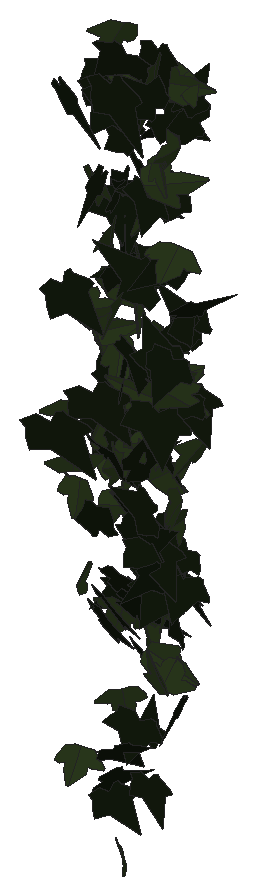
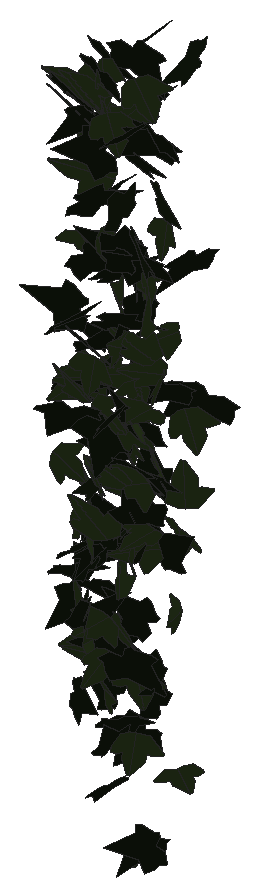
# SketchUp Ruby script. Lengths in inches.
U = 1.inch
M = Sketchup.active_model
def pt(a) = Geom::Point3d.new(a.map { |v| v * U })
def face(e, loops, mat)
  f = e.add_face(loops[0].map { |a| pt(a) })
  loops[1..].each { |l| e.add_face(l.map { |a| pt(a) }).erase! }
  f.material = f.back_material = mat if mat
  f
end
# faces: each face lists its corners as indices into pts; further lists are holes
def faces(e, pts, list, mat = nil) = list.each { |f| face(e, (f[0].is_a?(Array) ? f : [f]).map { |l| l.map { |i| pts[i] } }, mat) }
# xy, xz, yz: faces in a plane at the given z, y or x. An outline is a flat list of corners, or four numbers for a rectangle; further outlines are holes
def ring(l) = l.size == 4 ? [[l[0], l[1]], [l[2], l[1]], [l[2], l[3]], [l[0], l[3]]] : l.each_slice(2).to_a
def flat(e, list, mat, &to3) = list.each { |f| face(e, (f[0].is_a?(Array) ? f : [f]).map { |l| ring(l).map { |u, v| to3.(u, v) } }, mat) }
def xy(e, z, list, mat = nil) = flat(e, list, mat) { |x, y| [x, y, z] }
def xz(e, y, list, mat = nil) = flat(e, list, mat) { |x, z| [x, y, z] }
def yz(e, x, list, mat = nil) = flat(e, list, mat) { |y, z| [x, y, z] }
def lines(e, pts, list) = list.each { |a, b| e.add_line(pt(pts[a]), pt(pts[b])) }
# prism: a flat outline (further loops are holes) pulled along v
def prism(e, loops, v, mat = nil)
  f = face(e, loops, mat); d = Geom::Vector3d.new(v.map { |x| x * U })
  f.pushpull(f.normal.samedirection?(d) ? d.length : -d.length)
end
def box(e, o, s, mat = nil) = prism(e, [[o, [o[0] + s[0], o[1], o[2]], [o[0] + s[0], o[1] + s[1], o[2]], [o[0], o[1] + s[1], o[2]]]], [0, 0, s[2]], mat)
def at(x, y, z, deg = 0) = Geom::Transformation.translation(pt([x, y, z])) * Geom::Transformation.rotation(ORIGIN, Z_AXIS, deg.degrees)
def axes(o, x, y, z) = Geom::Transformation.new([*x, 0, *y, 0, *z, 0, *pt(o).to_a, 1])
def part(name) = M.definitions.add(name)
# library, detail: a bought-in or finely detailed component or shape, given as its bounding box
def library(name, o, s) = part(name).tap { |d| box(d.entities, o, s) }
def detail(e, o, s) = box(e.add_group.entities, o, s)
def put(e, d, t, mat = nil) = e.add_instance(d, t).tap { |i| i.material = mat if mat }
def group(e, t, mat = nil) = e.add_group.tap { |g| g.transformation = t; g.material = mat if mat }.entities
root = M.entities
M.materials.add("1026 AP 7946 SUNNY SIDE UP").color = [254, 231, 186]
M.materials.add("efeu1").color = [18, 25, 13]
M.materials.add("efeu2").color = [43, 57, 29]
c1 = part("ivyleaf_9")
p = [[1.54,2.16,1.25],[1.36,2.04,1.19],[-0.21,0.99,0.68],[-0.71,1.11,0.82],[-0.85,0.86,0.67],[-0.8,0.17,0.21],
  [-0.9,-0.01,0.1],[-0.67,-0.16,-0.02],[-0.08,-0.08,-0.05],[-0.03,-0.6,-0.4],[0.65,-0.88,-0.66],[0.83,-0.6,-0.49],
  [1.29,-0.42,-0.43],[1.8125,-0.07,-0.26],[1.21,0.44,0.15]]
faces(c1.entities,p,[[0,1,2,3,4,5,6,7,8,9,10,11,12,13,14]],"efeu1")
c2 = part("ivyleaf_10")
p = [[0,0.5,-0.03],[-0.0625,2.02,-0.43],[-0.19,2.01,-0.46],[-0.54,1.05,-0.29],[-0.52,0.625,-0.18],[-0.83,0.76,-0.28],
  [-1.16,0.64,-0.33],[-1.15,0.33,-0.24],[-0.77,-0.39,0.02],[-0.3,-0.51,0.16],[0.04,-0.48,0.23],[-0.02,2.01,-0.4375],
  [-0.06,2.01,-0.43],[0.04,-0.49,0.23],[0.67,-0.49,0.14],[1.38,0.36,-0.2],[1.375,0.51,-0.24],[0.81,0.65,-0.19],
  [0.62,0.59,-0.15],[0.6,1.09,-0.28],[0.5,1.23,-0.31]]
faces(c2.entities,p,[[0,1,2,3,4,5,6,7,8,9,10],[11,12,0,13,14,15,16,17,18,19,20]],"efeu2")
put(root,c1,axes([117.89,209.16,260.61],[-0.12502,-0.13654,-0.30499],[0.32147,0.21547,-0.1581],[0.39789,-0.21699,0.0319]),"1026 AP 7946 SUNNY SIDE UP")
put(root,c1,axes([118.01,209.3,267.36],[0.35139,-0.25579,-0.05878],[-0.08033,0.02908,-0.34919],[0.40368,0.22845,-0.01832]),"1026 AP 7946 SUNNY SIDE UP")
put(root,c1,axes([118.04,209.3,263.4],[0.10905,-0.2297,-0.2487],[-0.06595,0.23727,-0.24493],[0.51831,0.07852,0.02116]),"1026 AP 7946 SUNNY SIDE UP")
put(root,c1,axes([118.89,209.58,267.58],[0.16751,-0.3674,-0.0775],[-0.0277,0.07105,-0.39365],[0.58838,0.10794,0.00353]),"1026 AP 7946 SUNNY SIDE UP")
put(root,c1,axes([119.68,209.67,259.19],[0.02681,-0.30366,-0.03755],[0.03363,-0.03351,0.31249],[-0.4794,-0.01933,0.01982]),"1026 AP 7946 SUNNY SIDE UP")
put(root,c2,axes([117.7,209.92,260.55],[-0.22825,-0.27044,0.05167],[-0.01496,-0.05347,-0.31605],[0.43268,-0.14451,0.01633]),"1026 AP 7946 SUNNY SIDE UP")
put(root,c2,axes([118.62,210.08,262.89],[0.1701,-0.19875,0.2303],[0.12167,-0.21227,-0.23307],[0.45571,0.13086,-0.02374]),"1026 AP 7946 SUNNY SIDE UP")
put(root,c1,axes([118.25,209.89,261.01],[-0.0783,-0.2007,-0.24489],[0.20388,0.20421,-0.2054],[0.44317,-0.1294,0.05123]),"1026 AP 7946 SUNNY SIDE UP")
put(root,c2,axes([117.79,210.02,253.51],[0.28029,0.19308,-0.09406],[-0.07953,-0.07884,-0.27072],[-0.32705,0.18465,-0.01478]),"1026 AP 7946 SUNNY SIDE UP")
put(root,c1,axes([119.51,210.12,257.75],[-0.0668,0.06136,-0.27059],[0.09308,-0.25765,-0.07329],[-0.41433,-0.06777,0.02716]),"1026 AP 7946 SUNNY SIDE UP")
put(root,c1,axes([118.29,210.23,266.77],[-0.1118,-0.21782,0.17072],[-0.07074,-0.16088,-0.23692],[0.4257,-0.08394,0.00547]),"1026 AP 7946 SUNNY SIDE UP")
put(root,c1,axes([118.72,209.88,253.97],[0.27527,0.19906,0.05238],[0.06943,0.02727,-0.2725],[-0.31506,0.17993,-0.01429]),"1026 AP 7946 SUNNY SIDE UP")
put(root,c2,axes([119.66,210,255.55],[-0.30115,0.16584,-0.13563],[-0.13467,0.10306,0.26083],[0.3055,0.20891,-0.01872]),"1026 AP 7946 SUNNY SIDE UP")
put(root,c1,axes([119.43,210.22,260.87],[-0.19506,-0.27654,-0.09752],[0.07322,0.0811,-0.31164],[0.45293,-0.13221,0.00838]),"1026 AP 7946 SUNNY SIDE UP")
put(root,c2,axes([118.65,210.2,251.55],[-0.21172,0.17466,0.14632],[0.15877,-0.09978,0.22601],[0.31528,0.16753,-0.01555]),"1026 AP 7946 SUNNY SIDE UP")
put(root,c1,axes([119.29,210.2,258.15],[-0.07414,-0.25428,-0.16502],[0.10957,0.147,-0.26304],[0.45844,-0.07625,0.03618]),"1026 AP 7946 SUNNY SIDE UP")
put(root,c1,axes([119.47,210.03,267.21],[-0.12137,0.13688,0.25052],[-0.22034,0.19825,-0.16013],[-0.37822,-0.15941,0.0129]),"1026 AP 7946 SUNNY SIDE UP")
put(root,c2,axes([117.53,210.24,259.18],[-0.30253,-0.25451,-0.03509],[-0.05348,-0.01511,0.32808],[-0.39991,0.19456,-0.01733]),"1026 AP 7946 SUNNY SIDE UP")
put(root,c1,axes([118.77,210.4375,261.6875],[-0.02303,-0.23728,0.2184],[0.05144,-0.21356,-0.24363],[0.4991,0.01106,0.03519]),"1026 AP 7946 SUNNY SIDE UP")
put(root,c2,axes([119.13,210.28,261.125],[-0.13156,-0.04352,-0.27512],[-0.41464,-0.04835,0.09303],[-0.09359,0.27541,-0.02544]),"1026 AP 7946 SUNNY SIDE UP")
put(root,c1,axes([118.91,210.27,258.09],[-0.06697,0.0593,0.29108],[0.32388,-0.19339,0.07276],[0.31734,0.20989,-0.01283]),"1026 AP 7946 SUNNY SIDE UP")
put(root,c1,axes([119.625,210.36,261.95],[-0.39019,-0.07568,-0.12099],[0.19163,-0.00194,-0.26496],[0.10628,-0.27435,0.03352]),"1026 AP 7946 SUNNY SIDE UP")
put(root,c2,axes([118.77,210.34,259.96],[0.37069,-0.14453,0.05282],[0.05077,-0.04667,-0.28421],[0.23618,0.23688,-0.02181]),"1026 AP 7946 SUNNY SIDE UP")
put(root,c1,axes([118.83,210.42,254.35],[-0.23868,-0.21538,-0.01707],[0.03451,0.00327,-0.27093],[0.33777,-0.15253,0.01562]),"1026 AP 7946 SUNNY SIDE UP")
put(root,c1,axes([117.96,210.41,265.07],[-0.30032,0.07525,-0.25163],[0.3196,-0.14102,-0.20895],[-0.24471,-0.27652,0.03593]),"1026 AP 7946 SUNNY SIDE UP")
put(root,c1,axes([118.46,210.49,261.52],[-0.11282,-0.02764,-0.27999],[0.37587,-0.14206,-0.05099],[-0.20744,-0.24238,0.05988]),"1026 AP 7946 SUNNY SIDE UP")
put(root,c1,axes([118.98,210.07,259.69],[0.05149,0.07369,0.32786],[0.34732,0.23008,-0.07705],[-0.37756,0.22171,-0.02617]),"1026 AP 7946 SUNNY SIDE UP")
put(root,c1,axes([118.57,210.34,267.8],[0.18066,0.0622,-0.2606],[-0.31294,-0.15802,-0.13389],[-0.26511,0.22891,-0.01954]),"1026 AP 7946 SUNNY SIDE UP")
put(root,c2,axes([117.41,210.45,258.625],[0.3814,-0.10016,0.0848],[0.10439,-0.05542,-0.26947],[0.17575,0.25027,-0.02396]),"1026 AP 7946 SUNNY SIDE UP")
put(root,c1,axes([118.03,210.53,259.34],[0.43236,-0.16438,-0.07785],[0.13355,-0.0022,0.32735],[-0.25049,-0.2849,0.04017]),"1026 AP 7946 SUNNY SIDE UP")
put(root,c1,axes([118.94,210.6,264.97],[-0.08326,-0.25512,0.11036],[-0.02691,-0.10732,-0.26901],[0.43514,-0.05545,0.00448]),"1026 AP 7946 SUNNY SIDE UP")
put(root,c1,axes([119.01,210.54,263.21],[-0.23748,-0.30417,-0.03617],[-0.04349,-0.02351,0.34941],[-0.47918,0.15288,-0.01379]),"1026 AP 7946 SUNNY SIDE UP")
put(root,c2,axes([119.45,210.39,255.4],[0.40233,0.02742,-0.07135],[0.10307,0.03597,0.26377],[0.05611,-0.26267,0.02709]),"1026 AP 7946 SUNNY SIDE UP")
put(root,c2,axes([119.1,210.58,265.6875],[0.22542,-0.09301,0.23138],[0.30146,-0.11805,-0.17671],[0.23626,0.23937,0.00471]),"1026 AP 7946 SUNNY SIDE UP")
put(root,c2,axes([119.4,210.66,266.02],[-0.01006,0.0395,0.29127],[0.12409,-0.27131,0.03933],[0.43104,0.07903,-0.00452]),"1026 AP 7946 SUNNY SIDE UP")
put(root,c1,axes([117.92,210.39,258.01],[0.11424,-0.07137,0.30027],[-0.26332,0.23971,0.10473],[-0.39229,-0.18169,0.01714]),"1026 AP 7946 SUNNY SIDE UP")
put(root,c2,axes([117.65,210.28,256.84],[0.058,-0.03851,0.26789],[-0.18245,0.23348,0.0539],[-0.37128,-0.12075,0.01537]),"1026 AP 7946 SUNNY SIDE UP")
put(root,c2,axes([119.66,210.43,259.04],[0.21606,-0.27018,-0.13536],[-0.08771,0.11731,-0.31156],[0.46312,0.14826,0.00414]),"1026 AP 7946 SUNNY SIDE UP")
put(root,c1,axes([119.25,210.64,257.0625],[-0.36078,-0.1331,-0.0337],[0.06211,-0.00466,-0.2722],[0.20608,-0.23162,0.02304]),"1026 AP 7946 SUNNY SIDE UP")
put(root,c1,axes([118.93,210.59,253.1],[0.02293,-0.25363,-0.04997],[-0.00682,0.04689,-0.26144],[0.40556,0.01513,-0.00157]),"1026 AP 7946 SUNNY SIDE UP")
put(root,c2,axes([117.74,210.32,262.38],[0.00162,-0.04504,-0.30723],[0.23296,0.25956,-0.03837],[0.41264,-0.14636,0.02286]),"1026 AP 7946 SUNNY SIDE UP")
put(root,c2,axes([119.02,210.75,260],[-0.04851,0.03994,0.30529],[-0.06276,-0.29557,0.03506],[0.46562,-0.03568,0.03653]),"1026 AP 7946 SUNNY SIDE UP")
put(root,c2,axes([119.18,210.49,255.76],[0.17065,0.06931,0.28511],[0.41197,0.09192,-0.12921],[-0.17602,0.28232,-0.026]),"1026 AP 7946 SUNNY SIDE UP")
put(root,c2,axes([118.11,210.73,259.15],[-0.07921,0.10847,0.27956],[0.15036,-0.25343,0.12144],[0.43327,0.10778,0.00896]),"1026 AP 7946 SUNNY SIDE UP")
put(root,c1,axes([119.32,210.54,261.72],[-0.30706,-0.17895,0.10986],[0.10631,0.08528,0.27287],[-0.31069,0.20604,-0.01521]),"1026 AP 7946 SUNNY SIDE UP")
put(root,c1,axes([119.3,210.78,263.65],[-0.02249,0.00095,-0.29261],[0.04815,-0.28274,-0.00421],[-0.44403,-0.03071,0.01436]),"1026 AP 7946 SUNNY SIDE UP")
put(root,c1,axes([119.41,210.8,256.33],[-0.0398,-0.07219,0.25686],[-0.04798,-0.24837,-0.0786],[0.40595,-0.03643,0.0159]),"1026 AP 7946 SUNNY SIDE UP")
put(root,c2,axes([117.72,210.6,259.65],[0.27195,-0.21842,-0.0076],[0.02796,0.00627,0.28647],[-0.34244,-0.17295,0.01735]),"1026 AP 7946 SUNNY SIDE UP")
put(root,c2,axes([119.43,210.67,263.9375],[0.3982,0.10783,-0.08347],[-0.10153,-0.05588,-0.28271],[-0.18686,0.26014,-0.02427]),"1026 AP 7946 SUNNY SIDE UP")
put(root,c1,axes([119.52,210.77,254.8125],[-0.16421,0.07154,-0.25283],[0.26209,-0.18253,-0.12874],[-0.30558,-0.195,0.02545]),"1026 AP 7946 SUNNY SIDE UP")
put(root,c1,axes([119.58,210.79,257.33],[-0.24316,-0.23222,-0.00877],[0.0253,-0.00208,-0.28704],[0.36444,-0.15479,0.01407]),"1026 AP 7946 SUNNY SIDE UP")
put(root,c2,axes([118.18,210.71,261.45],[0.19102,0.26514,-0.10917],[-0.0497,-0.10361,-0.30073],[-0.4471,0.1248,-0.01321]),"1026 AP 7946 SUNNY SIDE UP")
put(root,c2,axes([118.27,210.84,260.54],[-0.06525,-0.1992,0.18117],[-0.05361,-0.17368,-0.21063],[0.41556,-0.05368,0.00127]),"1026 AP 7946 SUNNY SIDE UP")
put(root,c1,axes([119.53,210.87,261.02],[-0.32071,-0.17503,0.02733],[-0.01203,-0.03324,-0.2763],[0.27834,-0.20311,0.01955]),"1026 AP 7946 SUNNY SIDE UP")
put(root,c2,axes([119.4,210.6,261.11],[-0.25221,-0.16823,-0.26059],[0.31878,0.15231,-0.23679],[0.35406,-0.25697,0.02757]),"1026 AP 7946 SUNNY SIDE UP")
put(root,c1,axes([117.97,210.77,256.78],[0.32068,0.01393,-0.16905],[0.25102,0.04795,0.20876],[0.06413,-0.25738,0.02818]),"1026 AP 7946 SUNNY SIDE UP")
put(root,c1,axes([118.17,210.72,258.42],[0.45091,-0.14505,-0.03748],[-0.06549,-0.00374,-0.33031],[0.22552,0.28894,-0.02098]),"1026 AP 7946 SUNNY SIDE UP")
put(root,c1,axes([118.85,210.63,253.93],[-0.15939,-0.10615,0.21857],[0.21106,0.16537,0.15184],[-0.30861,0.16792,-0.00904]),"1026 AP 7946 SUNNY SIDE UP")
put(root,c2,axes([117.68,210.73,261.7],[-0.12905,0.26484,-0.02049],[-0.00297,-0.02298,-0.28564],[-0.41779,-0.08165,0.00836]),"1026 AP 7946 SUNNY SIDE UP")
put(root,c2,axes([119.06,210.63,265.24],[0.14067,0.01624,-0.33931],[0.47847,0.12771,0.09236],[0.20022,-0.3166,0.01769]),"1026 AP 7946 SUNNY SIDE UP")
put(root,c1,axes([119.45,210.97,257.8],[-0.15824,-0.2005,0.12695],[-0.05739,-0.12035,-0.23101],[0.36652,-0.10541,0.01863]),"1026 AP 7946 SUNNY SIDE UP")
put(root,c2,axes([119.35,210.98,258.33],[-0.00053,-0.02027,-0.27346],[-0.06297,-0.26231,0.01916],[-0.41366,0.03996,-0.00257]),"1026 AP 7946 SUNNY SIDE UP")
put(root,c2,axes([118.89,210.75,267.46],[0.01018,-0.3284,-0.10986],[0.03146,0.10497,-0.33707],[0.5411,0.00007,0.02166]),"1026 AP 7946 SUNNY SIDE UP")
put(root,c2,axes([118.76,210.85,266.68],[0.12519,-0.28067,0.02869],[0.00089,-0.03043,-0.30062],[0.44374,0.07924,-0.00749]),"1026 AP 7946 SUNNY SIDE UP")
put(root,c1,axes([118.43,210.71,265.96],[-0.29493,-0.01829,-0.2132],[-0.32651,0.01475,0.19272],[-0.00207,0.27883,-0.02253]),"1026 AP 7946 SUNNY SIDE UP")
put(root,c1,axes([117.84,210.91,259.8],[-0.36309,-0.09377,-0.08664],[0.13455,0.0106,-0.25576],[0.14459,-0.24534,0.02042]),"1026 AP 7946 SUNNY SIDE UP")
put(root,c2,axes([118.27,210.82,266.79],[0.22731,0.21344,0.10504],[-0.11283,-0.0728,0.26454],[0.35355,-0.16046,0.01689]),"1026 AP 7946 SUNNY SIDE UP")
put(root,c2,axes([117.57,210.76,264.76],[-0.34906,0.15718,0.04591],[-0.0782,0.00503,-0.27906],[-0.2443,-0.22619,0.02374]),"1026 AP 7946 SUNNY SIDE UP")
put(root,c2,axes([117.89,210.77,263.83],[0.03254,-0.30122,-0.10367],[0.02109,0.09987,-0.30983],[0.49807,0.01545,0.01989]),"1026 AP 7946 SUNNY SIDE UP")
put(root,c2,axes([118.34,210.95,262.5],[-0.08891,0.21599,-0.22142],[0.08243,-0.20971,-0.23123],[-0.47337,-0.07709,0.00132]),"1026 AP 7946 SUNNY SIDE UP")
put(root,c1,axes([118.66,211,258.1],[0.33461,-0.09722,-0.18923],[0.28017,-0.04844,0.23951],[-0.16672,-0.27654,0.0227]),"1026 AP 7946 SUNNY SIDE UP")
put(root,c1,axes([118.46,211,255.28],[0.18501,-0.17403,0.2102],[0.13848,-0.18652,-0.21626],[0.39955,0.14523,-0.02238]),"1026 AP 7946 SUNNY SIDE UP")
put(root,c1,axes([119.11,211.1,264.92],[-0.04385,-0.20893,-0.25074],[-0.0031,-0.24301,0.21477],[-0.50296,0.01971,0.02054]),"1026 AP 7946 SUNNY SIDE UP")
put(root,c1,axes([119.83,210.82,266.66],[-0.33326,0.1887,0.08839],[-0.12748,0.03583,-0.2909],[-0.29923,-0.22542,0.02548]),"1026 AP 7946 SUNNY SIDE UP")
put(root,c1,axes([117.89,210.81,252.4],[0.01889,-0.18114,-0.22089],[-0.02981,0.21257,-0.18575],[0.43911,0.02222,-0.00311]),"1026 AP 7946 SUNNY SIDE UP")
put(root,c2,axes([119.33,210.65,261.13],[-0.00602,-0.09291,0.326],[0.01359,0.31686,0.09764],[-0.5192,0.00937,-0.00122]),"1026 AP 7946 SUNNY SIDE UP")
put(root,c2,axes([117.82,210.7,261.77],[-0.05241,-0.06114,0.27893],[0.12202,0.26014,0.07179],[-0.41961,0.08328,-0.01396]),"1026 AP 7946 SUNNY SIDE UP")
put(root,c1,axes([119.01,211.08,257.625],[0.06887,-0.16706,0.22534],[0.08016,-0.21371,-0.17914],[0.4265,0.06714,-0.00272]),"1026 AP 7946 SUNNY SIDE UP")
put(root,c1,axes([117.95,211.08,263.75],[-0.08067,0.00295,-0.31149],[0.42226,-0.14054,-0.04918],[-0.21858,-0.2726,0.01996]),"1026 AP 7946 SUNNY SIDE UP")
put(root,c2,axes([118.6,211.12,264.33],[0.00225,-0.15635,0.24544],[0.04139,-0.23805,-0.1619],[0.44735,0.02281,0.01375]),"1026 AP 7946 SUNNY SIDE UP")
put(root,c2,axes([118.24,211.1,263.21],[0.00661,-0.01547,0.31027],[0.36966,-0.18863,-0.01446],[0.29722,0.23494,0.01108]),"1026 AP 7946 SUNNY SIDE UP")
put(root,c2,axes([118.94,210.78,260.66],[0.01461,-0.00687,-0.33471],[-0.34351,0.24044,-0.01027],[0.37821,0.21865,0.0036]),"1026 AP 7946 SUNNY SIDE UP")
put(root,c2,axes([118.65,210.85,256.58],[-0.10265,0.06452,0.25456],[-0.37947,0.06673,-0.08337],[-0.12968,-0.24635,0.04244]),"1026 AP 7946 SUNNY SIDE UP")
put(root,c2,axes([117.92,211.125,261.02],[0.171,-0.19655,0.21204],[0.11654,-0.19441,-0.23148],[0.43338,0.12983,-0.02142]),"1026 AP 7946 SUNNY SIDE UP")
put(root,c1,axes([118.04,210.77,263.14],[0.00315,-0.05086,-0.28498],[-0.16714,0.25567,-0.04778],[0.40898,0.10488,-0.01733]),"1026 AP 7946 SUNNY SIDE UP")
put(root,c1,axes([118.21,210.91,256.33],[0.38967,-0.03893,0.16487],[0.24137,-0.05128,-0.25768],[0.09479,0.29063,-0.02159]),"1026 AP 7946 SUNNY SIDE UP")
put(root,c2,axes([117.84,210.8,258.26],[-0.05245,-0.04439,-0.29334],[0.35256,0.17567,-0.05429],[0.28405,-0.22624,0.01322]),"1026 AP 7946 SUNNY SIDE UP")
put(root,c1,axes([117.88,210.93,260.625],[-0.20888,0.13966,0.23335],[0.26379,-0.15142,0.19734],[0.32342,0.2137,-0.01026]),"1026 AP 7946 SUNNY SIDE UP")
put(root,c2,axes([118.06,210.94,254.42],[-0.28719,-0.21957,-0.05603],[0.07126,0.03134,-0.29366],[0.348,-0.18762,0.01389]),"1026 AP 7946 SUNNY SIDE UP")
put(root,c1,axes([118.75,211.05,267.62],[-0.23615,-0.02728,-0.24469],[0.37403,0.00925,-0.15609],[0.03528,-0.28073,0.01697]),"1026 AP 7946 SUNNY SIDE UP")
put(root,c1,axes([118.36,211.1,259.95],[-0.48584,-0.04713,0.00166],[0.00421,-0.02999,-0.32067],[0.07404,-0.30753,0.02916]),"1026 AP 7946 SUNNY SIDE UP")
put(root,c2,axes([118.24,210.79,258.77],[0.1955,-0.06952,0.29817],[-0.31881,0.21044,0.14284],[-0.3435,-0.23489,0.03713]),"1026 AP 7946 SUNNY SIDE UP")
put(root,c1,axes([117.6,210.97,266.61],[-0.08443,-0.11368,-0.25472],[0.28536,0.17197,-0.12137],[0.31762,-0.18472,0.04134]),"1026 AP 7946 SUNNY SIDE UP")
put(root,c2,axes([117.96,211.14,258.13],[0.0234,-0.01552,0.26745],[0.32001,-0.16135,-0.02289],[0.25484,0.20404,0.00419]),"1026 AP 7946 SUNNY SIDE UP")
put(root,c1,axes([119.12,210.84,266.55],[0.05598,-0.06744,-0.28202],[-0.03844,0.27377,-0.07126],[0.44107,0.03242,0.02958]),"1026 AP 7946 SUNNY SIDE UP")
put(root,c1,axes([117.51,211.08,266.8],[-0.2569,-0.05891,-0.21817],[0.33458,0.02219,-0.17562],[0.08471,-0.26629,0.03198]),"1026 AP 7946 SUNNY SIDE UP")
put(root,c1,axes([118.73,210.99,258.05],[0.00841,-0.23033,-0.19506],[-0.00091,0.18806,-0.23623],[0.46754,0.00451,0.00305]),"1026 AP 7946 SUNNY SIDE UP")
put(root,c1,axes([117.51,211.16,255.9375],[0.16123,-0.16373,0.2214],[0.17797,-0.18379,-0.20009],[0.38703,0.15272,-0.00022]),"1026 AP 7946 SUNNY SIDE UP")
put(root,c2,axes([119.07,210.97,267.12],[-0.13377,0.00026,0.30586],[0.43381,0.11415,0.08201],[-0.17245,0.28697,-0.03095]),"1026 AP 7946 SUNNY SIDE UP")
put(root,c1,axes([119.49,211.06,262.25],[-0.39228,0.11411,0.01608],[-0.03796,-0.01696,-0.2815],[-0.17694,-0.24935,0.02474]),"1026 AP 7946 SUNNY SIDE UP")
put(root,c2,axes([119.22,211.08,267.27],[0.47082,-0.10001,-0.1504],[-0.23424,0.01037,-0.32327],[0.14883,0.33271,-0.03301]),"1026 AP 7946 SUNNY SIDE UP")
put(root,c1,axes([119.44,210.94,266.82],[-0.29915,0.19538,0.08655],[0.11912,-0.04149,0.27958],[0.31174,0.20334,-0.02377]),"1026 AP 7946 SUNNY SIDE UP")
put(root,c1,axes([119.59,211.12,262.24],[-0.19712,-0.27158,0.06078],[0.0219,0.06019,0.30824],[-0.43696,0.12553,-0.01197]),"1026 AP 7946 SUNNY SIDE UP")
put(root,c1,axes([118.06,211.32,265.09],[0.08478,-0.21629,0.26486],[0.07075,-0.25465,-0.23081],[0.52503,0.06924,-0.01167]),"1026 AP 7946 SUNNY SIDE UP")
put(root,c1,axes([119.39,210.91,262.6],[0.11663,0.25992,-0.11771],[0.03643,0.11369,0.279],[0.4459,-0.07727,0.008]),"1026 AP 7946 SUNNY SIDE UP")
put(root,c2,axes([118.78,211.27,258.14],[0.02608,-0.06985,-0.25821],[0.08199,-0.24476,0.07251],[-0.40022,-0.05469,-0.00197]),"1026 AP 7946 SUNNY SIDE UP")
put(root,c1,axes([117.33,211.23,255.5625],[0.15481,-0.13685,0.22109],[0.17621,-0.18422,-0.17443],[0.36049,0.14882,-0.00968]),"1026 AP 7946 SUNNY SIDE UP")
put(root,c2,axes([119.45,211.26,259.74],[-0.03105,-0.24156,0.19327],[-0.01014,-0.189,-0.25068],[0.48214,-0.01953,0.00717]),"1026 AP 7946 SUNNY SIDE UP")
put(root,c2,axes([117.78,211.18,267.68],[-0.22945,-0.26443,0.09724],[-0.04491,-0.09354,-0.31106],[0.44001,-0.14744,0.01896]),"1026 AP 7946 SUNNY SIDE UP")
put(root,c2,axes([118.8,211.32,256.29],[0.0682,-0.06532,0.29475],[0.21225,-0.2528,-0.08191],[0.4104,0.1416,-0.00662]),"1026 AP 7946 SUNNY SIDE UP")
put(root,c2,axes([118.46,211.15,266.74],[-0.27736,-0.23489,0.05339],[-0.02521,-0.0543,-0.30227],[0.37784,-0.17605,0.01903]),"1026 AP 7946 SUNNY SIDE UP")
put(root,c1,axes([117.85,211.2,264.25],[-0.31233,-0.16124,-0.19029],[0.25139,0.09351,-0.26196],[0.29088,-0.25395,0.02207]),"1026 AP 7946 SUNNY SIDE UP")
put(root,c2,axes([118.12,211.24,257.58],[-0.28298,0.13267,0.21512],[0.24066,-0.14198,0.22883],[0.30435,0.23562,0.01907]),"1026 AP 7946 SUNNY SIDE UP")
put(root,c2,axes([117.81,211.16,259.76],[-0.30147,0.04958,-0.24526],[0.3445,-0.09716,-0.20294],[-0.16693,-0.29006,0.02412]),"1026 AP 7946 SUNNY SIDE UP")
put(root,c1,axes([118.66,210.95,260.47],[0.17396,0.28255,0.03456],[0.03108,0.02655,-0.31232],[-0.44603,0.11205,-0.00828]),"1026 AP 7946 SUNNY SIDE UP")
put(root,c1,axes([118.65,211.2,259.52],[0.21961,-0.21297,0.01342],[-0.0056,-0.01933,-0.26211],[0.33557,0.13905,-0.01316]),"1026 AP 7946 SUNNY SIDE UP")
put(root,c1,axes([118.86,211.31,256.66],[0.00194,0.05721,0.32898],[-0.4121,-0.1875,0.03459],[0.29981,-0.2581,0.04541]),"1026 AP 7946 SUNNY SIDE UP")
put(root,c2,axes([119.09,211.17,261.1],[0.25186,-0.12794,-0.1753],[0.26567,-0.05172,0.20447],[-0.20216,-0.22735,0.05031]),"1026 AP 7946 SUNNY SIDE UP")
put(root,c1,axes([117.65,211.17,259.09],[0.38169,0.08528,0.03563],[-0.06274,0.01112,0.26401],[0.13007,-0.24488,0.02279]),"1026 AP 7946 SUNNY SIDE UP")
put(root,c2,axes([119.08,211.23,256.78],[-0.27271,0.15001,0.16836],[0.22155,-0.08435,0.23454],[0.26815,0.22225,-0.02255]),"1026 AP 7946 SUNNY SIDE UP")
put(root,c1,axes([117.64,210.95,252.49],[0.02789,0.18039,-0.20902],[-0.02316,0.20468,0.18641],[0.42746,-0.00068,0.02374]),"1026 AP 7946 SUNNY SIDE UP")
put(root,c1,axes([119.2,211.13,256.95],[0.39295,-0.08908,-0.06102],[-0.09997,-0.00422,-0.27215],[0.13473,0.25668,-0.02397]),"1026 AP 7946 SUNNY SIDE UP")
put(root,c2,axes([118.78,211.27,259.73],[0.29593,-0.22645,0.07331],[0.0504,-0.06739,-0.30317],[0.37043,0.19007,-0.01732]),"1026 AP 7946 SUNNY SIDE UP")
put(root,c1,axes([118.27,211.2,261.03],[0.14828,-0.24144,-0.10692],[-0.07321,0.09169,-0.26632],[0.40583,0.10476,-0.00898]),"1026 AP 7946 SUNNY SIDE UP")
put(root,c2,axes([117.66,211.14,262.4],[-0.24507,-0.03519,0.24739],[0.34641,0.0998,0.16282],[-0.16088,0.26851,-0.02628]),"1026 AP 7946 SUNNY SIDE UP")
put(root,c2,axes([117.62,211.22,262.99],[-0.28011,0.21373,0.0701],[0.08973,-0.03926,0.28579],[0.34049,0.18617,-0.01765]),"1026 AP 7946 SUNNY SIDE UP")
put(root,c1,axes([117.78,211.25,259.0625],[0.16333,-0.225,-0.04605],[-0.04301,0.03516,-0.25489],[0.35774,0.10695,-0.00962]),"1026 AP 7946 SUNNY SIDE UP")
put(root,c2,axes([117.85,211.21,255.95],[-0.42815,-0.04081,0.08271],[-0.118,-0.03988,-0.2825],[0.07889,-0.28113,0.02635]),"1026 AP 7946 SUNNY SIDE UP")
put(root,c1,axes([117.94,211.26,264.27],[0.1732,-0.05564,0.27195],[0.34251,-0.15046,-0.12703],[0.25109,0.24361,-0.0143]),"1026 AP 7946 SUNNY SIDE UP")
put(root,c1,axes([119.25,211.25,260.78],[-0.16219,-0.21295,-0.20311],[0.16419,0.16662,-0.2422],[0.42437,-0.14585,0.01608]),"1026 AP 7946 SUNNY SIDE UP")
put(root,c1,axes([118.32,211.4,262.94],[-0.34637,-0.07144,0.18427],[-0.24164,-0.09962,-0.23601],[0.18354,-0.26597,0.03701]),"1026 AP 7946 SUNNY SIDE UP")
put(root,c1,axes([117.88,211.05,264.48],[-0.18909,0.0616,-0.28814],[-0.37052,0.1518,0.13953],[0.2569,0.26428,-0.01085]),"1026 AP 7946 SUNNY SIDE UP")
put(root,c2,axes([118.79,211.24,261.83],[-0.42924,0.08664,0.00959],[-0.02611,-0.02329,-0.29385],[-0.13443,-0.27213,0.02643]),"1026 AP 7946 SUNNY SIDE UP")
put(root,c2,axes([118.2,211.23,259.72],[0.24451,-0.02766,-0.20473],[0.31467,0.0061,0.1606],[-0.0192,-0.25214,0.02485]),"1026 AP 7946 SUNNY SIDE UP")
put(root,c1,axes([117.92,211.43,266.81],[-0.04292,-0.29227,0.03737],[0.00125,-0.03817,-0.3026],[0.46342,-0.02697,0.00428]),"1026 AP 7946 SUNNY SIDE UP")
put(root,c2,axes([117.56,211.19,258.88],[0.14828,0.17096,0.17661],[0.14986,0.14177,-0.19997],[-0.34878,0.1336,-0.01084]),"1026 AP 7946 SUNNY SIDE UP")
put(root,c1,axes([118.6875,211.07,266.07],[-0.01057,0.22485,-0.20182],[-0.02566,0.19666,0.23275],[0.46954,0.01581,0.00817]),"1026 AP 7946 SUNNY SIDE UP")
put(root,c1,axes([117.96,211.36,256.3125],[0.06777,0.07088,-0.27075],[-0.22569,-0.22065,-0.08671],[-0.3644,0.14985,0.00335]),"1026 AP 7946 SUNNY SIDE UP")
put(root,c2,axes([118.54,211.31,256.83],[-0.37266,0.00896,-0.17192],[0.2572,-0.04734,-0.24214],[-0.05425,-0.286,0.03298]),"1026 AP 7946 SUNNY SIDE UP")
put(root,c2,axes([117.45,211.35,261.4375],[0.2972,0.1025,0.14975],[0.22088,0.04272,-0.21983],[-0.17034,0.23423,-0.02376]),"1026 AP 7946 SUNNY SIDE UP")
put(root,c2,axes([118.18,211.2,262.37],[0.03315,0.135,-0.23838],[0.04975,0.23,0.14209],[0.41934,-0.03796,0.00199]),"1026 AP 7946 SUNNY SIDE UP")
put(root,c2,axes([118.46,211.29,256.09],[-0.20027,-0.19593,-0.18959],[0.16968,0.1479,-0.23975],[0.38581,-0.16675,0.00703]),"1026 AP 7946 SUNNY SIDE UP")
put(root,c2,axes([118.46,211.4,258.72],[-0.37036,-0.0701,0.19132],[0.26248,0.08713,0.25195],[-0.16998,0.28727,-0.0278]),"1026 AP 7946 SUNNY SIDE UP")
put(root,c2,axes([118.45,211.3,255.45],[0.1687,-0.03914,0.26223],[-0.32622,0.15064,0.11473],[-0.24051,-0.23178,0.02832]),"1026 AP 7946 SUNNY SIDE UP")
